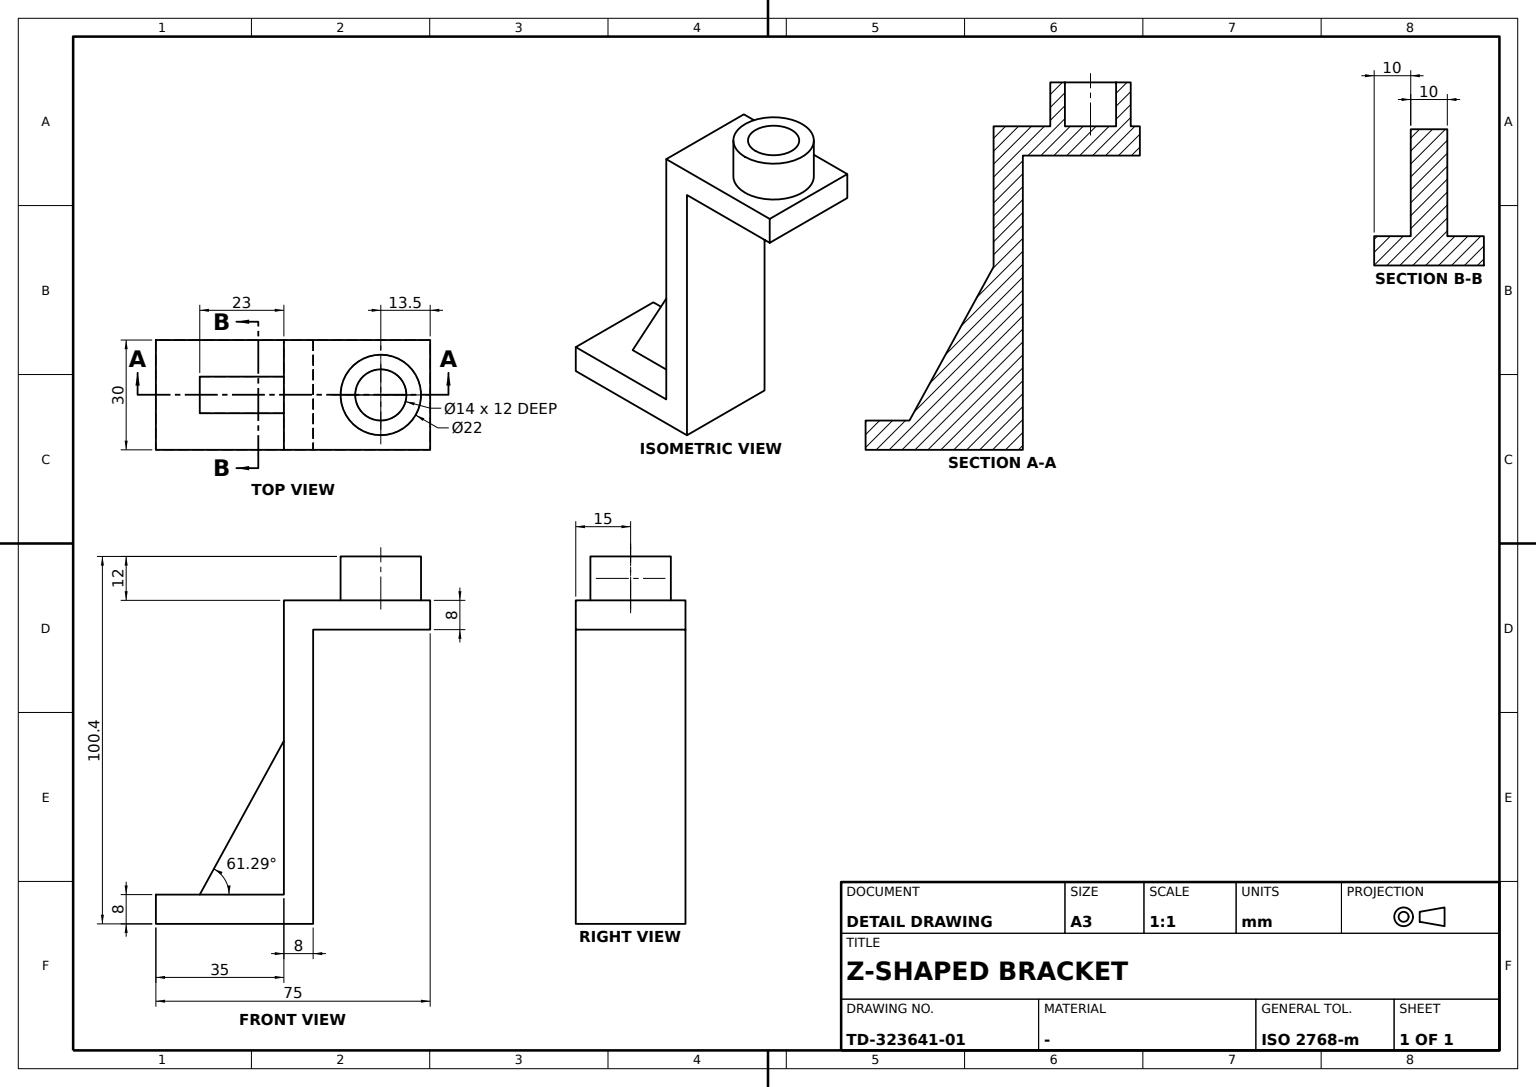
ISO-10303-21;
HEADER;
FILE_DESCRIPTION((''),'2;1');
FILE_NAME('','',(''),(''),'','','');
FILE_SCHEMA(('AUTOMOTIVE_DESIGN'));
ENDSEC;
DATA;
#1=APPLICATION_CONTEXT('');
#2=PRODUCT_CONTEXT('',#1,'mechanical');
#3=PRODUCT('','','',(#2));
#4=PRODUCT_DEFINITION_FORMATION('','',#3);
#5=PRODUCT_DEFINITION_CONTEXT('',#1,'design');
#6=PRODUCT_DEFINITION('','',#4,#5);
#7=PRODUCT_DEFINITION_SHAPE('','',#6);
#8=(LENGTH_UNIT()NAMED_UNIT(*)SI_UNIT(.MILLI.,.METRE.));
#9=(NAMED_UNIT(*)PLANE_ANGLE_UNIT()SI_UNIT($,.RADIAN.));
#10=(NAMED_UNIT(*)SI_UNIT($,.STERADIAN.)SOLID_ANGLE_UNIT());
#11=UNCERTAINTY_MEASURE_WITH_UNIT(LENGTH_MEASURE(0.005),#8,'distance_accuracy_value','');
#12=(GEOMETRIC_REPRESENTATION_CONTEXT(3)GLOBAL_UNCERTAINTY_ASSIGNED_CONTEXT((#11))GLOBAL_UNIT_ASSIGNED_CONTEXT((#8,#9,#10))REPRESENTATION_CONTEXT('',''));
#13=CARTESIAN_POINT('',(30.,-1.501339,44.199233));
#14=VERTEX_POINT('',#13);
#15=CARTESIAN_POINT('',(30.,38.498661,44.199233));
#16=VERTEX_POINT('',#15);
#17=CARTESIAN_POINT('',(30.,0.,44.199233));
#18=DIRECTION('',(0.,1.,0.));
#19=VECTOR('',#18,1000.);
#20=LINE('',#17,#19);
#21=EDGE_CURVE('',#14,#16,#20,.T.);
#22=ORIENTED_EDGE('',*,*,#21,.F.);
#23=CARTESIAN_POINT('',(30.,-1.501339,-36.199233));
#24=VERTEX_POINT('',#23);
#25=CARTESIAN_POINT('',(30.,-1.501339,0.));
#26=DIRECTION('',(0.,0.,1.));
#27=VECTOR('',#26,1000.);
#28=LINE('',#25,#27);
#29=EDGE_CURVE('',#24,#14,#28,.T.);
#30=ORIENTED_EDGE('',*,*,#29,.F.);
#31=CARTESIAN_POINT('',(30.,-36.501339,-36.199233));
#32=VERTEX_POINT('',#31);
#33=CARTESIAN_POINT('',(30.,0.,-36.199233));
#34=LINE('',#33,#19);
#35=EDGE_CURVE('',#32,#24,#34,.T.);
#36=ORIENTED_EDGE('',*,*,#35,.F.);
#37=CARTESIAN_POINT('',(30.,-36.501339,-44.199233));
#38=VERTEX_POINT('',#37);
#39=CARTESIAN_POINT('',(30.,-36.501339,0.));
#40=LINE('',#39,#27);
#41=EDGE_CURVE('',#38,#32,#40,.T.);
#42=ORIENTED_EDGE('',*,*,#41,.F.);
#43=CARTESIAN_POINT('',(30.,6.498661,-44.199233));
#44=VERTEX_POINT('',#43);
#45=CARTESIAN_POINT('',(30.,0.,-44.199233));
#46=DIRECTION('',(0.,-1.,0.));
#47=VECTOR('',#46,1000.);
#48=LINE('',#45,#47);
#49=EDGE_CURVE('',#44,#38,#48,.T.);
#50=ORIENTED_EDGE('',*,*,#49,.F.);
#51=CARTESIAN_POINT('',(30.,6.498661,36.199233));
#52=VERTEX_POINT('',#51);
#53=CARTESIAN_POINT('',(30.,6.498661,0.));
#54=DIRECTION('',(0.,0.,-1.));
#55=VECTOR('',#54,1000.);
#56=LINE('',#53,#55);
#57=EDGE_CURVE('',#52,#44,#56,.T.);
#58=ORIENTED_EDGE('',*,*,#57,.F.);
#59=CARTESIAN_POINT('',(30.,38.498661,36.199233));
#60=VERTEX_POINT('',#59);
#61=CARTESIAN_POINT('',(30.,0.,36.199233));
#62=LINE('',#61,#47);
#63=EDGE_CURVE('',#60,#52,#62,.T.);
#64=ORIENTED_EDGE('',*,*,#63,.F.);
#65=CARTESIAN_POINT('',(30.,38.498661,0.));
#66=LINE('',#65,#55);
#67=EDGE_CURVE('',#16,#60,#66,.T.);
#68=ORIENTED_EDGE('',*,*,#67,.F.);
#69=EDGE_LOOP('',(#22,#30,#36,#42,#50,#58,#64,#68));
#70=FACE_BOUND('',#69,.T.);
#71=CARTESIAN_POINT('',(30.,0.,0.));
#72=DIRECTION('',(1.,0.,0.));
#73=AXIS2_PLACEMENT_3D('',#71,#72,#18);
#74=PLANE('',#73);
#75=ADVANCED_FACE('',(#70),#74,.T.);
#76=CARTESIAN_POINT('',(20.,-1.501339,-36.199233));
#77=VERTEX_POINT('',#76);
#78=CARTESIAN_POINT('',(20.,-1.501339,5.800767));
#79=VERTEX_POINT('',#78);
#80=CARTESIAN_POINT('',(20.,-1.501339,0.));
#81=LINE('',#80,#27);
#82=EDGE_CURVE('',#77,#79,#81,.T.);
#83=ORIENTED_EDGE('',*,*,#82,.T.);
#84=CARTESIAN_POINT('',(20.,-24.501339,-36.199233));
#85=VERTEX_POINT('',#84);
#86=DIRECTION('',(0.,-0.480314623,-0.877096268));
#87=VECTOR('',#86,1000.);
#88=LINE('',#78,#87);
#89=EDGE_CURVE('',#79,#85,#88,.T.);
#90=ORIENTED_EDGE('',*,*,#89,.T.);
#91=CARTESIAN_POINT('',(20.,0.,-36.199233));
#92=LINE('',#91,#19);
#93=EDGE_CURVE('',#85,#77,#92,.T.);
#94=ORIENTED_EDGE('',*,*,#93,.T.);
#95=EDGE_LOOP('',(#83,#90,#94));
#96=FACE_BOUND('',#95,.T.);
#97=CARTESIAN_POINT('',(20.,0.,0.));
#98=AXIS2_PLACEMENT_3D('',#97,#72,#18);
#99=PLANE('',#98);
#100=ADVANCED_FACE('',(#96),#99,.T.);
#101=CARTESIAN_POINT('',(0.,-1.501339,44.199233));
#102=VERTEX_POINT('',#101);
#103=CARTESIAN_POINT('',(0.,38.498661,44.199233));
#104=VERTEX_POINT('',#103);
#105=CARTESIAN_POINT('',(0.,0.,44.199233));
#106=LINE('',#105,#19);
#107=EDGE_CURVE('',#102,#104,#106,.T.);
#108=ORIENTED_EDGE('',*,*,#107,.T.);
#109=CARTESIAN_POINT('',(0.,38.498661,36.199233));
#110=VERTEX_POINT('',#109);
#111=CARTESIAN_POINT('',(0.,38.498661,0.));
#112=LINE('',#111,#55);
#113=EDGE_CURVE('',#104,#110,#112,.T.);
#114=ORIENTED_EDGE('',*,*,#113,.T.);
#115=CARTESIAN_POINT('',(0.,6.498661,36.199233));
#116=VERTEX_POINT('',#115);
#117=CARTESIAN_POINT('',(0.,0.,36.199233));
#118=LINE('',#117,#47);
#119=EDGE_CURVE('',#110,#116,#118,.T.);
#120=ORIENTED_EDGE('',*,*,#119,.T.);
#121=CARTESIAN_POINT('',(0.,6.498661,-44.199233));
#122=VERTEX_POINT('',#121);
#123=CARTESIAN_POINT('',(0.,6.498661,0.));
#124=LINE('',#123,#55);
#125=EDGE_CURVE('',#116,#122,#124,.T.);
#126=ORIENTED_EDGE('',*,*,#125,.T.);
#127=CARTESIAN_POINT('',(0.,-36.501339,-44.199233));
#128=VERTEX_POINT('',#127);
#129=CARTESIAN_POINT('',(0.,0.,-44.199233));
#130=LINE('',#129,#47);
#131=EDGE_CURVE('',#122,#128,#130,.T.);
#132=ORIENTED_EDGE('',*,*,#131,.T.);
#133=CARTESIAN_POINT('',(0.,-36.501339,-36.199233));
#134=VERTEX_POINT('',#133);
#135=CARTESIAN_POINT('',(0.,-36.501339,0.));
#136=LINE('',#135,#27);
#137=EDGE_CURVE('',#128,#134,#136,.T.);
#138=ORIENTED_EDGE('',*,*,#137,.T.);
#139=CARTESIAN_POINT('',(0.,-1.501339,-36.199233));
#140=VERTEX_POINT('',#139);
#141=CARTESIAN_POINT('',(0.,0.,-36.199233));
#142=LINE('',#141,#19);
#143=EDGE_CURVE('',#134,#140,#142,.T.);
#144=ORIENTED_EDGE('',*,*,#143,.T.);
#145=CARTESIAN_POINT('',(0.,-1.501339,0.));
#146=LINE('',#145,#27);
#147=EDGE_CURVE('',#140,#102,#146,.T.);
#148=ORIENTED_EDGE('',*,*,#147,.T.);
#149=EDGE_LOOP('',(#108,#114,#120,#126,#132,#138,#144,#148));
#150=FACE_BOUND('',#149,.T.);
#151=CARTESIAN_POINT('',(0.,0.,0.));
#152=AXIS2_PLACEMENT_3D('',#151,#72,#18);
#153=PLANE('',#152);
#154=ADVANCED_FACE('',(#150),#153,.F.);
#155=ORIENTED_EDGE('',*,*,#67,.T.);
#156=VECTOR('',#72,1000.);
#157=LINE('',#109,#156);
#158=EDGE_CURVE('',#110,#60,#157,.T.);
#159=ORIENTED_EDGE('',*,*,#158,.F.);
#160=ORIENTED_EDGE('',*,*,#113,.F.);
#161=LINE('',#103,#156);
#162=EDGE_CURVE('',#104,#16,#161,.T.);
#163=ORIENTED_EDGE('',*,*,#162,.T.);
#164=EDGE_LOOP('',(#155,#159,#160,#163));
#165=FACE_BOUND('',#164,.T.);
#166=AXIS2_PLACEMENT_3D('',#103,#46,#54);
#167=PLANE('',#166);
#168=ADVANCED_FACE('',(#165),#167,.F.);
#169=CARTESIAN_POINT('',(26.,25.,56.199233));
#170=VERTEX_POINT('',#169);
#171=CARTESIAN_POINT('',(15.,25.,56.199233));
#172=AXIS2_PLACEMENT_3D('',#171,#26,#72);
#173=CIRCLE('',#172,11.);
#174=EDGE_CURVE('',#170,#170,#173,.T.);
#175=ORIENTED_EDGE('',*,*,#174,.F.);
#176=EDGE_LOOP('',(#175));
#177=FACE_BOUND('',#176,.T.);
#178=CARTESIAN_POINT('',(4.,25.,44.199233));
#179=VERTEX_POINT('',#178);
#180=CARTESIAN_POINT('',(15.,25.,44.199233));
#181=DIRECTION('',(-1.,0.,0.));
#182=AXIS2_PLACEMENT_3D('',#180,#54,#181);
#183=CIRCLE('',#182,11.);
#184=EDGE_CURVE('',#179,#179,#183,.F.);
#185=ORIENTED_EDGE('',*,*,#184,.T.);
#186=EDGE_LOOP('',(#185));
#187=FACE_BOUND('',#186,.T.);
#188=CARTESIAN_POINT('',(15.,25.,50.199233));
#189=AXIS2_PLACEMENT_3D('',#188,#26,#72);
#190=CYLINDRICAL_SURFACE('',#189,11.);
#191=ADVANCED_FACE('',(#177,#187),#190,.T.);
#192=ORIENTED_EDGE('',*,*,#89,.F.);
#193=CARTESIAN_POINT('',(10.,-1.501339,5.800767));
#194=VERTEX_POINT('',#193);
#195=CARTESIAN_POINT('',(0.,-1.501339,5.800767));
#196=VECTOR('',#181,1000.);
#197=LINE('',#195,#196);
#198=EDGE_CURVE('',#79,#194,#197,.T.);
#199=ORIENTED_EDGE('',*,*,#198,.T.);
#200=CARTESIAN_POINT('',(10.,-24.501339,-36.199233));
#201=VERTEX_POINT('',#200);
#202=LINE('',#193,#87);
#203=EDGE_CURVE('',#194,#201,#202,.T.);
#204=ORIENTED_EDGE('',*,*,#203,.T.);
#205=CARTESIAN_POINT('',(15.,-24.501339,-36.199233));
#206=LINE('',#205,#196);
#207=EDGE_CURVE('',#85,#201,#206,.T.);
#208=ORIENTED_EDGE('',*,*,#207,.F.);
#209=EDGE_LOOP('',(#192,#199,#204,#208));
#210=FACE_BOUND('',#209,.T.);
#211=CARTESIAN_POINT('',(15.,-1.501339,5.800767));
#212=DIRECTION('',(0.,0.877096268,-0.480314623));
#213=AXIS2_PLACEMENT_3D('',#211,#212,#86);
#214=PLANE('',#213);
#215=ADVANCED_FACE('',(#210),#214,.F.);
#216=LINE('',#133,#156);
#217=EDGE_CURVE('',#134,#32,#216,.T.);
#218=ORIENTED_EDGE('',*,*,#217,.F.);
#219=ORIENTED_EDGE('',*,*,#137,.F.);
#220=LINE('',#127,#156);
#221=EDGE_CURVE('',#128,#38,#220,.T.);
#222=ORIENTED_EDGE('',*,*,#221,.T.);
#223=ORIENTED_EDGE('',*,*,#41,.T.);
#224=EDGE_LOOP('',(#218,#219,#222,#223));
#225=FACE_BOUND('',#224,.T.);
#226=AXIS2_PLACEMENT_3D('',#127,#18,#26);
#227=PLANE('',#226);
#228=ADVANCED_FACE('',(#225),#227,.F.);
#229=ORIENTED_EDGE('',*,*,#184,.F.);
#230=EDGE_LOOP('',(#229));
#231=FACE_BOUND('',#230,.T.);
#232=ORIENTED_EDGE('',*,*,#162,.F.);
#233=ORIENTED_EDGE('',*,*,#107,.F.);
#234=LINE('',#101,#156);
#235=EDGE_CURVE('',#102,#14,#234,.T.);
#236=ORIENTED_EDGE('',*,*,#235,.T.);
#237=ORIENTED_EDGE('',*,*,#21,.T.);
#238=EDGE_LOOP('',(#232,#233,#236,#237));
#239=FACE_BOUND('',#238,.T.);
#240=AXIS2_PLACEMENT_3D('',#101,#54,#18);
#241=PLANE('',#240);
#242=ADVANCED_FACE('',(#231,#239),#241,.F.);
#243=CARTESIAN_POINT('',(22.,25.,56.199233));
#244=VERTEX_POINT('',#243);
#245=CIRCLE('',#172,7.);
#246=EDGE_CURVE('',#244,#244,#245,.T.);
#247=ORIENTED_EDGE('',*,*,#246,.F.);
#248=EDGE_LOOP('',(#247));
#249=FACE_BOUND('',#248,.T.);
#250=ORIENTED_EDGE('',*,*,#174,.T.);
#251=EDGE_LOOP('',(#250));
#252=FACE_BOUND('',#251,.T.);
#253=CARTESIAN_POINT('',(0.,0.,56.199233));
#254=AXIS2_PLACEMENT_3D('',#253,#26,#72);
#255=PLANE('',#254);
#256=ADVANCED_FACE('',(#249,#252),#255,.T.);
#257=ORIENTED_EDGE('',*,*,#246,.T.);
#258=EDGE_LOOP('',(#257));
#259=FACE_BOUND('',#258,.T.);
#260=CARTESIAN_POINT('',(8.,25.,44.199233));
#261=VERTEX_POINT('',#260);
#262=CIRCLE('',#182,7.);
#263=EDGE_CURVE('',#261,#261,#262,.F.);
#264=ORIENTED_EDGE('',*,*,#263,.F.);
#265=EDGE_LOOP('',(#264));
#266=FACE_BOUND('',#265,.T.);
#267=CYLINDRICAL_SURFACE('',#189,7.);
#268=ADVANCED_FACE('',(#259,#266),#267,.F.);
#269=LINE('',#115,#156);
#270=EDGE_CURVE('',#116,#52,#269,.T.);
#271=ORIENTED_EDGE('',*,*,#270,.F.);
#272=ORIENTED_EDGE('',*,*,#119,.F.);
#273=ORIENTED_EDGE('',*,*,#158,.T.);
#274=ORIENTED_EDGE('',*,*,#63,.T.);
#275=EDGE_LOOP('',(#271,#272,#273,#274));
#276=FACE_BOUND('',#275,.T.);
#277=AXIS2_PLACEMENT_3D('',#109,#26,#46);
#278=PLANE('',#277);
#279=ADVANCED_FACE('',(#276),#278,.F.);
#280=ORIENTED_EDGE('',*,*,#35,.T.);
#281=LINE('',#139,#156);
#282=EDGE_CURVE('',#77,#24,#281,.T.);
#283=ORIENTED_EDGE('',*,*,#282,.F.);
#284=ORIENTED_EDGE('',*,*,#93,.F.);
#285=ORIENTED_EDGE('',*,*,#207,.T.);
#286=CARTESIAN_POINT('',(10.,-1.501339,-36.199233));
#287=VERTEX_POINT('',#286);
#288=CARTESIAN_POINT('',(10.,0.,-36.199233));
#289=LINE('',#288,#19);
#290=EDGE_CURVE('',#201,#287,#289,.T.);
#291=ORIENTED_EDGE('',*,*,#290,.T.);
#292=EDGE_CURVE('',#140,#287,#281,.T.);
#293=ORIENTED_EDGE('',*,*,#292,.F.);
#294=ORIENTED_EDGE('',*,*,#143,.F.);
#295=ORIENTED_EDGE('',*,*,#217,.T.);
#296=EDGE_LOOP('',(#280,#283,#284,#285,#291,#293,#294,#295));
#297=FACE_BOUND('',#296,.T.);
#298=AXIS2_PLACEMENT_3D('',#133,#54,#18);
#299=PLANE('',#298);
#300=ADVANCED_FACE('',(#297),#299,.F.);
#301=ORIENTED_EDGE('',*,*,#57,.T.);
#302=LINE('',#121,#156);
#303=EDGE_CURVE('',#122,#44,#302,.T.);
#304=ORIENTED_EDGE('',*,*,#303,.F.);
#305=ORIENTED_EDGE('',*,*,#125,.F.);
#306=ORIENTED_EDGE('',*,*,#270,.T.);
#307=EDGE_LOOP('',(#301,#304,#305,#306));
#308=FACE_BOUND('',#307,.T.);
#309=AXIS2_PLACEMENT_3D('',#115,#46,#54);
#310=PLANE('',#309);
#311=ADVANCED_FACE('',(#308),#310,.F.);
#312=ORIENTED_EDGE('',*,*,#203,.F.);
#313=CARTESIAN_POINT('',(10.,-1.501339,0.));
#314=LINE('',#313,#27);
#315=EDGE_CURVE('',#287,#194,#314,.T.);
#316=ORIENTED_EDGE('',*,*,#315,.F.);
#317=ORIENTED_EDGE('',*,*,#290,.F.);
#318=EDGE_LOOP('',(#312,#316,#317));
#319=FACE_BOUND('',#318,.T.);
#320=CARTESIAN_POINT('',(10.,0.,0.));
#321=AXIS2_PLACEMENT_3D('',#320,#72,#18);
#322=PLANE('',#321);
#323=ADVANCED_FACE('',(#319),#322,.F.);
#324=ORIENTED_EDGE('',*,*,#131,.F.);
#325=ORIENTED_EDGE('',*,*,#303,.T.);
#326=ORIENTED_EDGE('',*,*,#49,.T.);
#327=ORIENTED_EDGE('',*,*,#221,.F.);
#328=EDGE_LOOP('',(#324,#325,#326,#327));
#329=FACE_BOUND('',#328,.T.);
#330=AXIS2_PLACEMENT_3D('',#121,#26,#46);
#331=PLANE('',#330);
#332=ADVANCED_FACE('',(#329),#331,.F.);
#333=ORIENTED_EDGE('',*,*,#263,.T.);
#334=EDGE_LOOP('',(#333));
#335=FACE_BOUND('',#334,.T.);
#336=ADVANCED_FACE('',(#335),#241,.F.);
#337=ORIENTED_EDGE('',*,*,#292,.T.);
#338=ORIENTED_EDGE('',*,*,#315,.T.);
#339=ORIENTED_EDGE('',*,*,#198,.F.);
#340=ORIENTED_EDGE('',*,*,#82,.F.);
#341=ORIENTED_EDGE('',*,*,#282,.T.);
#342=ORIENTED_EDGE('',*,*,#29,.T.);
#343=ORIENTED_EDGE('',*,*,#235,.F.);
#344=ORIENTED_EDGE('',*,*,#147,.F.);
#345=EDGE_LOOP('',(#337,#338,#339,#340,#341,#342,#343,#344));
#346=FACE_BOUND('',#345,.T.);
#347=AXIS2_PLACEMENT_3D('',#139,#18,#26);
#348=PLANE('',#347);
#349=ADVANCED_FACE('',(#346),#348,.F.);
#350=CLOSED_SHELL('',(#75,#100,#154,#168,#191,#215,#228,#242,#256,#268,#279,#300,#311,#323,#332,#336,#349));
#351=MANIFOLD_SOLID_BREP('',#350);
#352=ADVANCED_BREP_SHAPE_REPRESENTATION('',(#351),#12);
#353=SHAPE_DEFINITION_REPRESENTATION(#7,#352);
ENDSEC;
END-ISO-10303-21;
